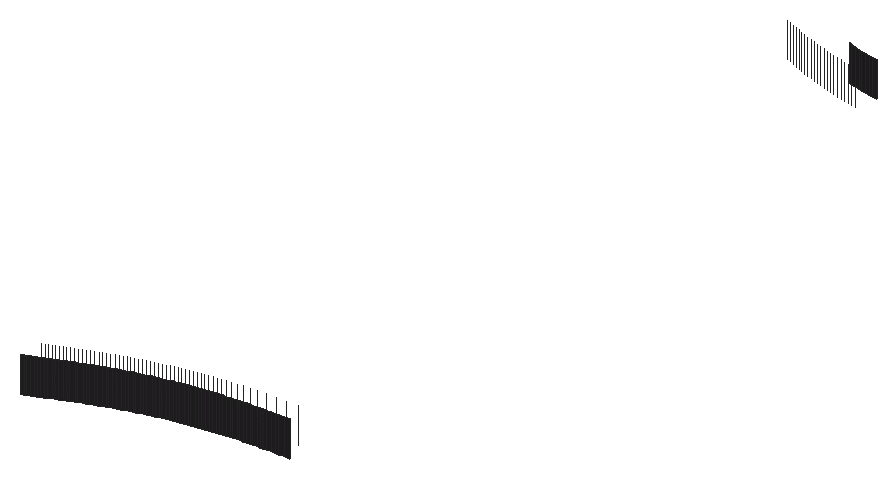
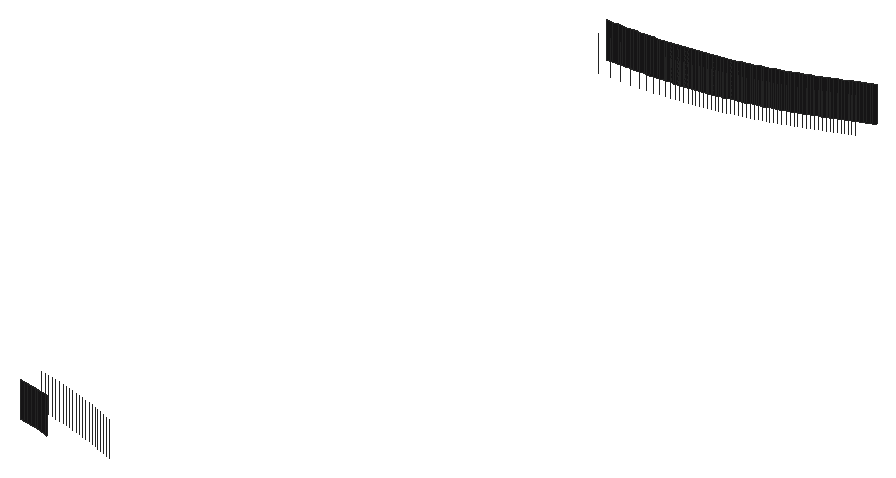
# SketchUp Ruby script. Lengths in inches.
U = 1.inch
M = Sketchup.active_model
def pt(a) = Geom::Point3d.new(a.map { |v| v * U })
def face(e, loops, mat)
  f = e.add_face(loops[0].map { |a| pt(a) })
  loops[1..].each { |l| e.add_face(l.map { |a| pt(a) }).erase! }
  f.material = f.back_material = mat if mat
  f
end
# faces: each face lists its corners as indices into pts; further lists are holes
def faces(e, pts, list, mat = nil) = list.each { |f| face(e, (f[0].is_a?(Array) ? f : [f]).map { |l| l.map { |i| pts[i] } }, mat) }
# xy, xz, yz: faces in a plane at the given z, y or x. An outline is a flat list of corners, or four numbers for a rectangle; further outlines are holes
def ring(l) = l.size == 4 ? [[l[0], l[1]], [l[2], l[1]], [l[2], l[3]], [l[0], l[3]]] : l.each_slice(2).to_a
def flat(e, list, mat, &to3) = list.each { |f| face(e, (f[0].is_a?(Array) ? f : [f]).map { |l| ring(l).map { |u, v| to3.(u, v) } }, mat) }
def xy(e, z, list, mat = nil) = flat(e, list, mat) { |x, y| [x, y, z] }
def xz(e, y, list, mat = nil) = flat(e, list, mat) { |x, z| [x, y, z] }
def yz(e, x, list, mat = nil) = flat(e, list, mat) { |y, z| [x, y, z] }
def lines(e, pts, list) = list.each { |a, b| e.add_line(pt(pts[a]), pt(pts[b])) }
# prism: a flat outline (further loops are holes) pulled along v
def prism(e, loops, v, mat = nil)
  f = face(e, loops, mat); d = Geom::Vector3d.new(v.map { |x| x * U })
  f.pushpull(f.normal.samedirection?(d) ? d.length : -d.length)
end
def box(e, o, s, mat = nil) = prism(e, [[o, [o[0] + s[0], o[1], o[2]], [o[0] + s[0], o[1] + s[1], o[2]], [o[0], o[1] + s[1], o[2]]]], [0, 0, s[2]], mat)
def at(x, y, z, deg = 0) = Geom::Transformation.translation(pt([x, y, z])) * Geom::Transformation.rotation(ORIGIN, Z_AXIS, deg.degrees)
def axes(o, x, y, z) = Geom::Transformation.new([*x, 0, *y, 0, *z, 0, *pt(o).to_a, 1])
def part(name) = M.definitions.add(name)
# library, detail: a bought-in or finely detailed component or shape, given as its bounding box
def library(name, o, s) = part(name).tap { |d| box(d.entities, o, s) }
def detail(e, o, s) = box(e.add_group.entities, o, s)
def put(e, d, t, mat = nil) = e.add_instance(d, t).tap { |i| i.material = mat if mat }
def group(e, t, mat = nil) = e.add_group.tap { |g| g.transformation = t; g.material = mat if mat }.entities
root = M.entities
M.materials.add("Marble_07_1K").color = [36, 34, 36]
xz(root,775.2,[[358.29,18,358.38,19]],"Marble_07_1K")
xz(root,775.21,[[358.47,18,358.5625,19]],"Marble_07_1K")
xz(root,775.22,[[358.65,18,358.74,19]],"Marble_07_1K")
xz(root,775.23,[[358.84,18,358.93,19],[358.93,18,359.02,19],[359.02,18,359.12,19]],"Marble_07_1K")
xz(root,775.24,[[359.22,18,359.34,19],[359.34,18,359.46,19]],"Marble_07_1K")
xz(root,775.25,[[359.6,18,359.76,19]],"Marble_07_1K")
p = [[353.29,773.8,18],[353.36,773.83,18],[353.36,773.83,19],[353.29,773.8,19],[353.4375,773.86,18],[353.4375,773.86,19],
  [353.51,773.89,18],[353.51,773.89,19],[353.58,773.92,18],[353.58,773.92,19],[353.65,773.95,18],[353.65,773.95,19],
  [353.73,773.98,18],[353.73,773.98,19],[353.8,774.01,18],[353.8,774.01,19],[353.875,774.04,18],[353.875,774.04,19],
  [353.95,774.08,18],[353.95,774.08,19],[354.03,774.11,18],[354.03,774.11,19],[354.11,774.14,18],[354.11,774.14,19],
  [354.19,774.18,18],[354.19,774.18,19],[354.27,774.21,18],[354.27,774.21,19],[354.35,774.24,18],[354.35,774.24,19],
  [354.4375,774.28,18],[354.4375,774.28,19],[354.52,774.3125,18],[354.52,774.3125,19],[354.61,774.35,18],[354.61,774.35,19],
  [354.69,774.38,18],[354.69,774.38,19],[354.78,774.41,18],[354.78,774.41,19],[354.86,774.44,18],[354.86,774.44,19],
  [354.95,774.47,18],[354.95,774.47,19],[355.03,774.51,18],[355.03,774.51,19],[355.12,774.54,18],[355.12,774.54,19],
  [355.2,774.5625,18],[355.2,774.5625,19],[355.29,774.59,18],[355.29,774.59,19],[355.375,774.62,18],[355.375,774.62,19],
  [355.46,774.65,18],[355.46,774.65,19],[355.55,774.68,18],[355.55,774.68,19],[355.63,774.7,18],[355.63,774.7,19],
  [355.72,774.73,18],[355.72,774.73,19],[355.81,774.75,18],[355.81,774.75,19],[355.89,774.78,18],[355.89,774.78,19],
  [355.98,774.8,18],[355.98,774.8,19],[356.07,774.82,18],[356.07,774.82,19],[356.16,774.85,18],[356.16,774.85,19],
  [356.24,774.87,18],[356.24,774.87,19],[356.33,774.89,18],[356.33,774.89,19],[356.42,774.91,18],[356.42,774.91,19],
  [356.51,774.93,18],[356.51,774.93,19],[356.6,774.95,18],[356.6,774.95,19],[356.68,774.97,18],[356.68,774.97,19],
  [356.77,774.98,18],[356.77,774.98,19],[356.86,775,18],[356.86,775,19],[356.95,775.02,18],[356.95,775.02,19],
  [357.04,775.04,18],[357.04,775.04,19],[357.125,775.05,18],[357.125,775.05,19],[357.22,775.07,18],[357.22,775.07,19],
  [357.3,775.08,18],[357.3,775.08,19],[357.39,775.09,18],[357.39,775.09,19],[357.48,775.11,18],[357.48,775.11,19],
  [357.57,775.12,18],[357.57,775.12,19],[357.66,775.13,18],[357.66,775.13,19],[357.75,775.14,18],[357.75,775.14,19],
  [357.84,775.15,18],[357.84,775.15,19],[357.93,775.16,18],[357.93,775.16,19],[358.02,775.17,18],[358.02,775.17,19],
  [358.11,775.18,18],[358.11,775.18,19],[358.2,775.1875,18],[358.2,775.1875,19],[358.29,775.2,18],[358.29,775.2,19],
  [358.38,775.2,18],[358.47,775.21,18],[358.47,775.21,19],[358.38,775.2,19],[358.5625,775.21,18],[358.65,775.22,18],
  [358.65,775.22,19],[358.5625,775.21,19],[358.74,775.22,18],[358.84,775.23,18],[358.84,775.23,19],[358.74,775.22,19],
  [359.12,775.23,18],[359.22,775.24,18],[359.22,775.24,19],[359.12,775.23,19],[359.46,775.24,18],[359.6,775.25,18],
  [359.6,775.25,19],[359.46,775.24,19],[359.64,796.03,18],[359.52,796.06,18],[359.52,796.06,19],[359.64,796.03,19],
  [359.76,796.01,18],[359.76,796.01,19],[359.17,796.14,18],[359.05,796.16,18],[359.05,796.16,19],[359.17,796.14,19],
  [359.28,796.11,18],[359.28,796.11,19],[359.4,796.08,18],[359.4,796.08,19],[358.93,796.19,18],[358.82,796.23,18],
  [358.82,796.23,19],[358.93,796.19,19],[353.35,774.48,18],[353.35,774.48,19],[353.42,774.51,18],[353.42,774.51,19],
  [353.5,774.54,18],[353.5,774.54,19],[353.57,774.57,18],[353.57,774.57,19],[353.64,774.6,18],[353.64,774.6,19],
  [353.72,774.63,18],[353.72,774.63,19],[353.8,774.67,18],[353.8,774.67,19],[353.88,774.7,18],[353.88,774.7,19],
  [353.96,774.73,18],[353.96,774.73,19],[354.04,774.77,18],[354.04,774.77,19],[354.13,774.8,18],[354.13,774.8,19],
  [354.21,774.84,18],[354.21,774.84,19],[354.3,774.875,18],[354.3,774.875,19],[354.39,774.91,18],[354.39,774.91,19],
  [354.48,774.94,18],[354.48,774.94,19],[354.57,774.98,18],[354.57,774.98,19],[354.65,775.01,18],[354.65,775.01,19],
  [354.74,775.04,18],[354.74,775.04,19],[354.83,775.07,18],[354.83,775.07,19],[354.92,775.11,18],[354.92,775.11,19],
  [355.01,775.14,18],[355.01,775.14,19],[355.1,775.17,18],[355.1,775.17,19],[355.19,775.2,18],[355.19,775.2,19],
  [355.28,775.22,18],[355.28,775.22,19],[355.37,775.25,18],[355.37,775.25,19],[355.46,775.28,18],[355.46,775.28,19],
  [355.55,775.31,18],[355.55,775.31,19],[355.64,775.33,18],[355.64,775.33,19],[355.73,775.36,18],[355.73,775.36,19],
  [355.82,775.38,18],[355.82,775.38,19],[355.92,775.41,18],[355.92,775.41,19],[356.01,775.43,18],[356.01,775.43,19],
  [356.1,775.45,18],[356.1,775.45,19],[356.19,775.48,18],[356.19,775.48,19],[356.28,775.5,18],[356.28,775.5,19],
  [356.375,775.52,18],[356.375,775.52,19],[356.47,775.54,18],[356.47,775.54,19],[356.56,775.56,18],[356.56,775.56,19],
  [356.65,775.58,18],[356.65,775.58,19],[356.75,775.59,18],[356.75,775.59,19],[356.84,775.61,18],[356.84,775.61,19],
  [356.94,775.63,18],[356.94,775.63,19],[357.03,775.65,18],[357.03,775.65,19],[357.13,775.66,18],[357.13,775.66,19],
  [357.24,775.68,18],[357.24,775.68,19],[357.35,775.7,18],[357.35,775.7,19],[357.46,775.71,18],[357.46,775.71,19],
  [357.58,775.73,18],[357.58,775.73,19],[357.71,775.74,18],[357.71,775.74,19],[357.86,775.76,18],[357.86,775.76,19],
  [358.02,775.78,18],[358.02,775.78,19],[358.2,775.79,18],[358.2,775.79,19],[358.4,775.81,18],[358.4,775.81,19],
  [358.64,775.82,18],[358.64,775.82,19],[358.9,775.84,18],[358.9,775.84,19],[359.2,775.84,18],[359.2,775.84,19],
  [359.53,775.85,18],[359.53,775.85,19],[359.64,795.42,18],[359.64,795.42,19],[359.52,795.44,18],[359.52,795.44,19],
  [359.39,795.47,18],[359.39,795.47,19],[359.27,795.49,18],[359.27,795.49,19],[359.15,795.52,18],[359.15,795.52,19],
  [359.02,795.55,18],[359.02,795.55,19],[358.9,795.58,18],[358.9,795.58,19],[358.78,795.61,18],[358.78,795.61,19],
  [358.66,795.64,18],[358.66,795.64,19],[358.54,795.68,18],[358.54,795.68,19],[358.41,795.71,18],[358.41,795.71,19],
  [358.29,795.75,18],[358.29,795.75,19],[358.17,795.79,18],[358.17,795.79,19],[358.05,795.83,18],[358.05,795.83,19],
  [357.93,795.87,18],[357.93,795.87,19],[357.8125,795.91,18],[357.8125,795.91,19],[357.69,795.95,18],[357.69,795.95,19],
  [357.58,796,18],[357.58,796,19],[357.46,796.04,18],[357.46,796.04,19],[357.34,796.09,18],[357.34,796.09,19],
  [357.22,796.14,18],[357.22,796.14,19],[357.11,796.18,18],[357.11,796.18,19]]
faces(root,p,[[0,1,2,3],[1,4,5,2],[4,6,7,5],[6,8,9,7],[8,10,11,9],[10,12,13,11],[12,14,15,13],[14,16,17,15],
  [16,18,19,17],[18,20,21,19],[20,22,23,21],[22,24,25,23],[24,26,27,25],[26,28,29,27],[28,30,31,29],[30,32,33,31],
  [32,34,35,33],[34,36,37,35],[36,38,39,37],[38,40,41,39],[40,42,43,41],[42,44,45,43],[44,46,47,45],[46,48,49,47],
  [48,50,51,49],[50,52,53,51],[52,54,55,53],[54,56,57,55],[56,58,59,57],[58,60,61,59],[60,62,63,61],[62,64,65,63],
  [64,66,67,65],[66,68,69,67],[68,70,71,69],[70,72,73,71],[72,74,75,73],[74,76,77,75],[76,78,79,77],[78,80,81,79],
  [80,82,83,81],[82,84,85,83],[84,86,87,85],[86,88,89,87],[88,90,91,89],[90,92,93,91],[92,94,95,93],[94,96,97,95],
  [96,98,99,97],[98,100,101,99],[100,102,103,101],[102,104,105,103],[104,106,107,105],[106,108,109,107],[108,110,111,109],[110,112,113,111],
  [112,114,115,113],[114,116,117,115],[116,118,119,117],[120,121,122,123],[124,125,126,127],[128,129,130,131],[132,133,134,135],[136,137,138,139],
  [140,141,142,143],[144,140,143,145],[146,147,148,149],[150,146,149,151],[152,150,151,153],[141,152,153,142],[154,155,156,157],[147,154,157,148]],"Marble_07_1K")
lines(root,p,[[158,159],[160,161],[162,163],[164,165],[166,167],[168,169],[170,171],[172,173],[174,175],[176,177],[178,179],[180,181],
  [182,183],[184,185],[186,187],[188,189],[190,191],[192,193],[194,195],[196,197],[198,199],[200,201],[202,203],[204,205],
  [206,207],[208,209],[210,211],[212,213],[214,215],[216,217],[218,219],[220,221],[222,223],[224,225],[226,227],[228,229],
  [230,231],[232,233],[234,235],[236,237],[238,239],[240,241],[242,243],[244,245],[246,247],[248,249],[250,251],[252,253],
  [254,255],[256,257],[258,259],[260,261],[262,263],[264,265],[266,267],[268,269],[270,271],[272,273],[274,275],[276,277],
  [278,279],[280,281],[282,283],[284,285],[286,287],[288,289],[290,291],[292,293],[294,295],[296,297],[298,299],[300,301],
  [302,303],[304,305],[306,307],[308,309],[310,311],[312,313],[314,315]])
